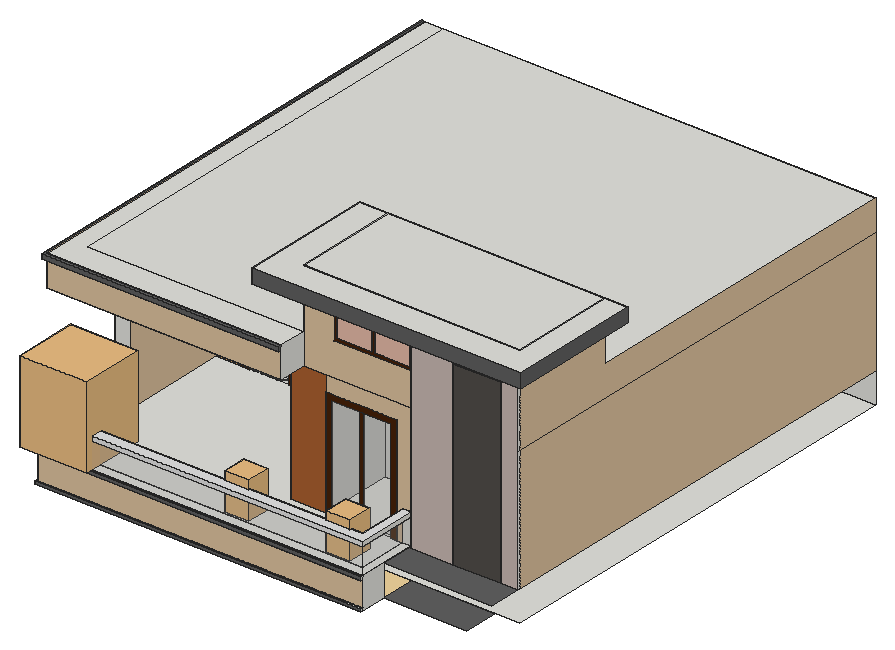
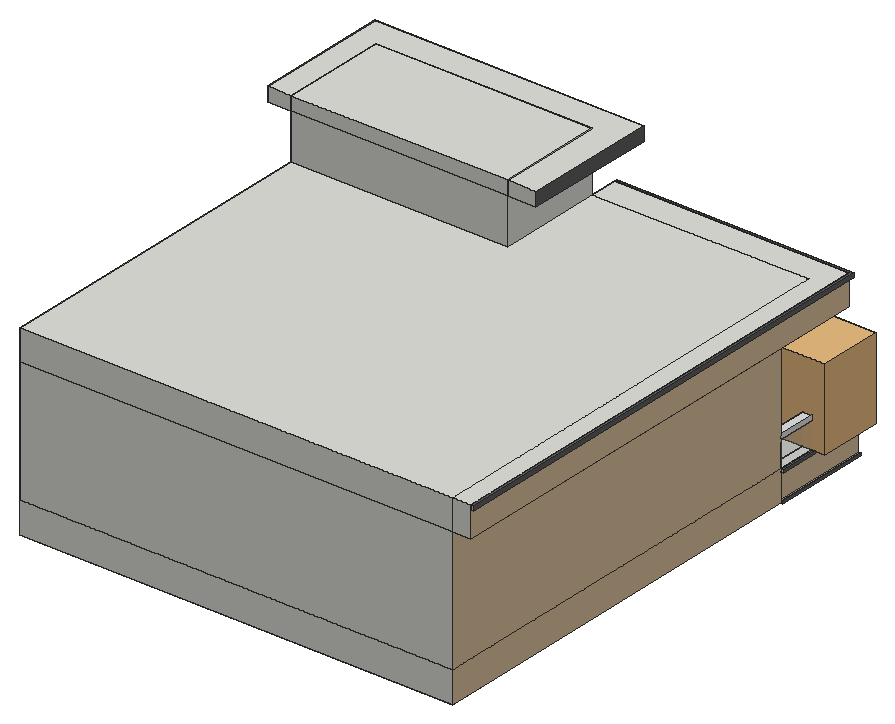
# SketchUp Ruby script. Lengths in inches.
U = 1.inch
M = Sketchup.active_model
def pt(a) = Geom::Point3d.new(a.map { |v| v * U })
def face(e, loops, mat)
  f = e.add_face(loops[0].map { |a| pt(a) })
  loops[1..].each { |l| e.add_face(l.map { |a| pt(a) }).erase! }
  f.material = f.back_material = mat if mat
  f
end
# faces: each face lists its corners as indices into pts; further lists are holes
def faces(e, pts, list, mat = nil) = list.each { |f| face(e, (f[0].is_a?(Array) ? f : [f]).map { |l| l.map { |i| pts[i] } }, mat) }
# xy, xz, yz: faces in a plane at the given z, y or x. An outline is a flat list of corners, or four numbers for a rectangle; further outlines are holes
def ring(l) = l.size == 4 ? [[l[0], l[1]], [l[2], l[1]], [l[2], l[3]], [l[0], l[3]]] : l.each_slice(2).to_a
def flat(e, list, mat, &to3) = list.each { |f| face(e, (f[0].is_a?(Array) ? f : [f]).map { |l| ring(l).map { |u, v| to3.(u, v) } }, mat) }
def xy(e, z, list, mat = nil) = flat(e, list, mat) { |x, y| [x, y, z] }
def xz(e, y, list, mat = nil) = flat(e, list, mat) { |x, z| [x, y, z] }
def yz(e, x, list, mat = nil) = flat(e, list, mat) { |y, z| [x, y, z] }
def lines(e, pts, list) = list.each { |a, b| e.add_line(pt(pts[a]), pt(pts[b])) }
# prism: a flat outline (further loops are holes) pulled along v
def prism(e, loops, v, mat = nil)
  f = face(e, loops, mat); d = Geom::Vector3d.new(v.map { |x| x * U })
  f.pushpull(f.normal.samedirection?(d) ? d.length : -d.length)
end
def box(e, o, s, mat = nil) = prism(e, [[o, [o[0] + s[0], o[1], o[2]], [o[0] + s[0], o[1] + s[1], o[2]], [o[0], o[1] + s[1], o[2]]]], [0, 0, s[2]], mat)
def at(x, y, z, deg = 0) = Geom::Transformation.translation(pt([x, y, z])) * Geom::Transformation.rotation(ORIGIN, Z_AXIS, deg.degrees)
def axes(o, x, y, z) = Geom::Transformation.new([*x, 0, *y, 0, *z, 0, *pt(o).to_a, 1])
def part(name) = M.definitions.add(name)
# library, detail: a bought-in or finely detailed component or shape, given as its bounding box
def library(name, o, s) = part(name).tap { |d| box(d.entities, o, s) }
def detail(e, o, s) = box(e.add_group.entities, o, s)
def put(e, d, t, mat = nil) = e.add_instance(d, t).tap { |i| i.material = mat if mat }
def group(e, t, mat = nil) = e.add_group.tap { |g| g.transformation = t; g.material = mat if mat }.entities
root = M.entities
M.materials.add("Generic").color = [222, 194, 159]
M.materials.add("Generic\#1").color = [230, 172, 103]
M.materials.add("Generic\#2").color = [241, 212, 157]
M.materials.add("[Color M01]").color = [226, 226, 226]
M.materials.add("[Color M07]").color = [96, 96, 96]
M.materials.add("[Mirror 02]").color = [229, 186, 167]
M.materials.add("[Roofing Shingles GAF Estates]").color = [81, 77, 74]
M.materials.add("[Stone Marble]").color = [201, 185, 179]
M.materials.add("[Translucent Glass Gray]").color = [175, 175, 175]
M.materials["[Translucent Glass Gray]"].alpha = 0.14
M.materials.add("[Wood Cherry Original]").color = [170, 96, 47]
M.materials.add("[Wood Veneer 01]").color = [71, 34, 9]
c1 = library("Group3\#1",[-238.15,54.18,0],[46.4,43.96,56.68])
c2 = part("Group\#3")
xy(c2.entities,0,[[0,0,140.875,6.8125]])
xy(c2.entities,105.3125,[[0,0,140.875,6.8125]])
xz(c2.entities,0,[[10.8,0,48.56,94.52],[52.56,0,88.32,94.52],[92.32,0,130.08,94.52]],"[Translucent Glass Gray]")
xz(c2.entities,0,[[0,0,10.8,0,10.8,94.52,48.56,94.52,48.56,0,52.56,0,52.56,94.52,88.32,94.52,88.32,0,92.32,0,92.32,94.52,130.08,94.52,130.08,0,140.875,0,140.875,105.3125,0,105.3125]],"[Wood Veneer 01]")
xz(c2.entities,6.8125,[[0,0,140.875,105.3125]],"[Translucent Glass Gray]")
yz(c2.entities,0,[[0,0,6.8125,105.3125]])
yz(c2.entities,140.875,[[0,0,6.8125,105.3125]])
c3 = library("Raised potted plant",[1.65,0,0],[13.63,13.63,20.73])
c4 = library("Tlon Light 450 Ceiling 152 006",[-8.86,-8.86,-3.78],[17.72,17.72,3.56])
xy(root,269.9375,[[217.875,91.73,217.875,228.48,35.6875,228.48,35.6875,125.1,20.1875,125.1,20.1875,523.73,440.1875,523.73,440.1875,91.73]])
xy(root,269.9375,[[[20.1875,32.23,20.1875,125.1,35.6875,125.1,35.6875,228.48,217.875,228.48,217.875,91.73,230.1875,91.73,230.1875,32.23],[58.88,55.42,194.68,205.29]],[230.1875,32.23,335.12,91.73]],"Generic\#2")
xy(root,269.9375,[[18.3125,30.41,18.3125,125.1,20.1875,125.1,20.1875,32.23,230.1875,32.23,230.1875,30.41],[230.1875,30.41,335.12,32.23],[335.12,57.98,416.1875,91.73]],"[Color M07]")
xy(root,269.9375,[[67.93,55.42,68.93,205.29],[78.5,55.42,79.5,205.29],[89.06,55.42,90.06,205.29],[99.62,55.42,100.62,205.29],[110.18,55.42,111.18,205.29],
  [120.75,55.42,121.75,205.29],[131.31,55.42,132.31,205.29],[141.87,55.42,142.87,205.29],[152.43,55.42,153.43,205.29],[163,55.42,164,205.29],
  [173.56,55.42,174.56,205.29],[184.12,55.42,185.12,205.29]],"[Wood Cherry Original]")
xy(root,272.5,[[230.1875,30.41,335.12,32.23]])
xy(root,272.5,[[18.3125,30.41,230.1875,30.41,230.1875,32.23,20.1875,32.23,20.1875,125.1,18.3125,125.1]],"[Color M07]")
xy(root,297,[[17.5625,30.41,17.5625,125.1,20.1875,125.1,20.1875,32.23,335.12,32.23,335.12,30.41]],"[Color M07]")
xy(root,299.875,[[20.1875,32.23,20.1875,125.1,29.125,125.1,29.125,42.6,326.8,42.6,326.8,91.73,335.12,91.73,335.12,32.23],[29.125,42.6,326.8,42.6,326.8,91.73,320.89,91.73,320.89,163.35,252.08,163.35,252.08,91.73,217.875,91.73,217.875,228.48,199.08,228.48,199.08,425.29,58.21,425.29,58.21,228.48,35.6875,228.48,35.6875,125.1,29.125,125.1],[337.01,89.1,377.69,91.73],[423.56,89.1,440.1875,91.73],[217.875,91.73,217.875,228.48,199.08,228.48,199.08,425.29,58.21,425.29,58.21,228.48,35.6875,228.48,35.6875,125.1,20.1875,125.1,20.1875,523.73,440.1875,523.73,440.1875,91.73,320.89,91.73,320.89,163.35,252.08,163.35,252.08,91.73]])
xy(root,299.875,[[17.5625,30.41,335.12,30.41,335.12,32.23,20.1875,32.23,20.1875,125.1,17.5625,125.1],[335.12,57.98,440.1875,57.98,440.1875,89.1,423.56,89.1,423.56,91.73,377.69,91.73,377.69,89.1,337.01,89.1,337.01,91.73,335.12,91.73]],"[Color M07]")
xy(root,325.25,[[20.1875,32.23,20.1875,125.1,29.125,125.1,29.125,42.6,326.8,42.6,326.8,91.73,335.12,91.73,335.12,32.23]])
xy(root,329.875,[[20.1875,32.23,335.12,32.23,335.12,91.73,326.8,91.73,326.8,42.6,29.125,42.6,29.125,125.1,20.1875,125.1]],"[Color M01]")
xy(root,404.625,[[252.08,91.73,320.89,163.35]])
xy(root,405.1875,[[58.21,228.48,199.08,425.29]])
xy(root,419.3125,[[52.42,86.71,65.86,206.5],[66.86,86.71,80.3125,206.5],[81.3125,86.71,94.76,206.5],[95.76,86.71,109.21,206.5],[110.21,86.71,123.66,206.5],
  [124.66,86.71,138.1,206.5],[139.1,86.71,152.55,206.5],[153.55,86.71,167,206.5],[168,86.71,181.45,206.5],[182.45,86.71,194.9,206.5]],"[Wood Cherry Original]")
xy(root,419.875,[[2.8125,228.48,20.1875,523.73]])
xy(root,419.875,[[[2.8125,64.73,2.8125,228.48,20.1875,228.48,20.1875,125.1,35.6875,125.1,35.6875,228.48,217.875,228.48,217.875,91.73,230.1875,91.73,230.1875,64.73],[52.42,86.71,194.9,206.5]]],"Generic\#2")
xy(root,419.875,[[65.86,86.71,66.86,206.5],[80.3125,86.71,81.3125,206.5],[94.76,86.71,95.76,206.5],[109.21,86.71,110.21,206.5],[123.66,86.71,124.66,206.5],
  [138.1,86.71,139.1,206.5],[152.55,86.71,153.55,206.5],[167,86.71,168,206.5],[181.45,86.71,182.45,206.5]],"[Wood Cherry Original]")
xy(root,445.25,[[0,64.73,2.8125,523.73]],"Generic")
xy(root,445.3125,[[0,61.91,230.1875,64.73]],"Generic")
xy(root,449.8125,[[2.8125,64.73,230.1875,64.73,230.1875,91.73,20.1875,91.73,20.1875,523.73,2.8125,523.73],[20.1875,91.73,230.1875,91.73,230.1875,194.66,440.1875,194.66,440.1875,523.73,20.1875,523.73]])
xy(root,449.8125,[[0,61.91,230.1875,61.91,230.1875,64.73,2.8125,64.73,2.8125,523.73,0,523.73]],"[Color M07]")
xy(root,455.39,[[262.97,91.73,296.69,119.1],[299.88,91.73,333.6,119.1]])
xy(root,474.97,[[377.69,89.1,423.56,91.73]])
xy(root,478.32,[[262.97,91.73,296.69,119.1],[299.88,91.73,333.6,119.1]])
xy(root,493.5625,[[337.01,89.1,440.1875,91.73],[230.1875,91.73,440.1875,194.66]])
xy(root,493.5625,[[202.5625,64.1,202.5625,194.66,230.1875,194.66,230.1875,91.73,337.01,91.73,337.01,89.1,440.1875,89.1,440.1875,194.66,462.9375,194.66,462.9375,64.1]],"[Wood Cherry Original]")
xy(root,507.375,[[202.5625,64.1,462.9375,64.1,462.9375,194.66,440.1875,194.66,440.1875,91.73,230.1875,91.73,230.1875,194.66,202.5625,194.66],[230.1875,91.73,440.1875,194.66]])
xz(root,30.41,[[18.3125,269.9375,335.12,272.5],[17.5625,297,335.12,299.875]],"[Color M07]")
xz(root,32.23,[[20.1875,269.9375,335.12,272.5],[20.1875,297,335.12,299.875]])
xz(root,32.23,[[20.1875,272.5,335.12,297]],"Generic")
xz(root,32.23,[[20.1875,325.25,335.12,329.875]],"[Color M01]")
xz(root,32.23,[[20.1875,299.875,335.12,325.25]],"[Translucent Glass Gray]")
xz(root,42.6,[[29.125,325.25,326.8,329.875]])
xz(root,42.6,[[29.125,299.875,326.8,325.25]],"[Translucent Glass Gray]")
xz(root,61.91,[[0,445.3125,230.1875,449.8125]],"[Color M07]")
xz(root,64.1,[[202.5625,493.5625,462.9375,507.375]],"[Color M07]")
xz(root,64.73,[[2.8125,419.875,230.1875,445.3125],[0,445.25,2.8125,445.3125],[2.8125,445.3125,230.1875,449.8125]],"Generic")
xz(root,86.71,[[52.42,419.3125,65.86,419.875],[66.86,419.3125,80.3125,419.875],[81.3125,419.3125,94.76,419.875],[95.76,419.3125,109.21,419.875],[110.21,419.3125,123.66,419.875],
  [124.66,419.3125,138.1,419.875],[139.1,419.3125,152.55,419.875],[153.55,419.3125,167,419.875],[168,419.3125,181.45,419.875],[182.45,419.3125,194.9,419.875]],"[Wood Cherry Original]")
xz(root,89.1,[[337.01,299.875,377.69,299.875,377.69,474.97,423.56,474.97,423.56,299.875,440.1875,299.875,440.1875,493.5625,337.01,493.5625]],"[Stone Marble]")
xz(root,91.73,[[326.8,299.875,335.12,325.25],[337.01,299.875,337.01,493.5625,440.1875,493.5625,440.1875,299.875,423.56,299.875,423.56,474.97,377.69,474.97,377.69,299.875],[377.69,299.875,423.56,474.97],[326.8,325.25,335.12,329.875],[230.1875,493.5625,440.1875,507.375]])
xz(root,91.73,[[320.89,299.875,326.8,299.875,326.8,329.875,335.12,329.875,335.12,299.875,337.01,299.875,337.01,419.875,252.08,419.875,252.08,404.625,320.89,404.625],[230.1875,419.875,337.01,419.875,337.01,451.98,259.5625,451.98,259.5625,481.73,337.01,481.73,337.01,493.5625,230.1875,493.5625]],"Generic")
xz(root,91.73,[[262.97,455.39,296.69,478.32],[299.88,455.39,333.6,478.32]],"[Mirror 02]")
xz(root,91.73,[[217.875,299.875,252.08,419.875]],"[Wood Cherry Original]")
xz(root,91.73,[[[259.5625,451.98,337.01,481.73],[299.88,455.39,333.6,478.32],[262.97,455.39,296.69,478.32]]],"[Wood Veneer 01]")
xz(root,119.1,[[262.97,455.39,296.69,478.32],[299.88,455.39,333.6,478.32]])
xz(root,125.1,[[18.3125,269.9375,20.1875,272.5],[17.5625,297,20.1875,299.875],[29.125,299.875,35.6875,299.875,35.6875,419.875,20.1875,419.875,20.1875,329.875,29.125,329.875]])
xz(root,163.35,[[252.08,299.875,320.89,404.625]])
xz(root,194.66,[[230.1875,449.8125,440.1875,493.5625],[202.5625,493.5625,230.1875,507.375],[230.1875,493.5625,440.1875,507.375],[440.1875,493.5625,462.9375,507.375]])
xz(root,206.5,[[52.42,419.3125,65.86,419.875],[66.86,419.3125,80.3125,419.875],[81.3125,419.3125,94.76,419.875],[95.76,419.3125,109.21,419.875],[110.21,419.3125,123.66,419.875],
  [124.66,419.3125,138.1,419.875],[139.1,419.3125,152.55,419.875],[153.55,419.3125,167,419.875],[168,419.3125,181.45,419.875],[182.45,419.3125,194.9,419.875]])
xz(root,228.48,[[35.6875,299.875,58.21,299.875,58.21,405.1875,199.08,405.1875,199.08,299.875,217.875,299.875,217.875,419.875,35.6875,419.875]],"Generic\#1")
xz(root,425.29,[[58.21,299.875,199.08,405.1875]])
xz(root,523.73,[[20.1875,269.9375,440.1875,299.875],[20.1875,299.875,440.1875,419.875],[2.8125,419.875,20.1875,449.8125],[20.1875,419.875,440.1875,449.8125]])
xz(root,523.73,[[0,445.25,2.8125,449.8125]],"Generic")
yz(root,0,[[64.73,445.25,64.73,445.3125,61.91,445.3125,61.91,449.8125,523.73,449.8125,523.73,445.25]],"[Color M07]")
yz(root,2.8125,[[64.73,419.875,523.73,445.25],[64.73,445.25,523.73,449.8125]],"Generic")
yz(root,17.5625,[[30.41,297,125.1,299.875]],"[Color M07]")
yz(root,18.3125,[[30.41,269.9375,125.1,272.5]],"[Color M07]")
yz(root,20.1875,[[32.23,269.9375,125.1,272.5],[32.23,297,125.1,299.875]])
yz(root,20.1875,[[125.1,269.9375,523.73,299.875],[32.23,272.5,125.1,297],[125.1,299.875,523.73,419.875]],"Generic")
yz(root,20.1875,[[32.23,325.25,125.1,329.875]],"[Color M01]")
yz(root,20.1875,[[32.23,299.875,125.1,325.25]],"[Translucent Glass Gray]")
yz(root,29.125,[[42.6,325.25,125.1,329.875]])
yz(root,29.125,[[42.6,299.875,125.1,325.25]],"[Translucent Glass Gray]")
yz(root,35.6875,[[125.1,299.875,228.48,419.875]],"Generic")
yz(root,52.42,[[86.71,419.3125,103.12,419.875],[103.12,419.3125,206.5,419.875]],"[Wood Cherry Original]")
yz(root,58.21,[[228.48,299.875,425.29,405.1875]])
yz(root,65.86,[[86.71,419.3125,206.5,419.875]],"[Wood Cherry Original]")
yz(root,66.86,[[86.71,419.3125,206.5,419.875]],"[Wood Cherry Original]")
yz(root,80.3125,[[86.71,419.3125,206.5,419.875]],"[Wood Cherry Original]")
yz(root,81.3125,[[86.71,419.3125,206.5,419.875]],"[Wood Cherry Original]")
yz(root,94.76,[[86.71,419.3125,206.5,419.875]],"[Wood Cherry Original]")
yz(root,95.76,[[86.71,419.3125,206.5,419.875]],"[Wood Cherry Original]")
yz(root,109.21,[[86.71,419.3125,206.5,419.875]],"[Wood Cherry Original]")
yz(root,110.21,[[86.71,419.3125,206.5,419.875]],"[Wood Cherry Original]")
yz(root,123.66,[[86.71,419.3125,206.5,419.875]],"[Wood Cherry Original]")
yz(root,124.66,[[86.71,419.3125,206.5,419.875]],"[Wood Cherry Original]")
yz(root,138.1,[[86.71,419.3125,206.5,419.875]],"[Wood Cherry Original]")
yz(root,139.1,[[86.71,419.3125,206.5,419.875]],"[Wood Cherry Original]")
yz(root,152.55,[[86.71,419.3125,206.5,419.875]],"[Wood Cherry Original]")
yz(root,153.55,[[86.71,419.3125,206.5,419.875]],"[Wood Cherry Original]")
yz(root,167,[[86.71,419.3125,206.5,419.875]],"[Wood Cherry Original]")
yz(root,168,[[86.71,419.3125,206.5,419.875]],"[Wood Cherry Original]")
yz(root,181.45,[[86.71,419.3125,206.5,419.875]],"[Wood Cherry Original]")
yz(root,182.45,[[86.71,419.3125,206.5,419.875]],"[Wood Cherry Original]")
yz(root,194.9,[[86.71,419.3125,206.5,419.875]],"[Wood Cherry Original]")
yz(root,199.08,[[228.48,299.875,425.29,405.1875]])
yz(root,202.5625,[[64.1,493.5625,194.66,507.375]],"[Color M07]")
yz(root,217.875,[[91.73,299.875,228.48,419.875]],"[Wood Cherry Original]")
yz(root,230.1875,[[64.73,419.875,91.73,449.8125],[91.73,449.8125,194.66,493.5625],[91.73,493.5625,194.66,507.375]])
yz(root,230.1875,[[61.91,445.3125,64.73,449.8125]],"[Color M07]")
yz(root,252.08,[[91.73,299.875,163.35,404.625]])
yz(root,262.97,[[91.73,455.39,119.1,478.32]])
yz(root,296.69,[[91.73,455.39,119.1,478.32]])
yz(root,299.88,[[91.73,455.39,119.1,478.32]])
yz(root,320.89,[[91.73,299.875,163.35,404.625]])
yz(root,326.8,[[42.6,325.25,91.73,329.875]])
yz(root,326.8,[[42.6,299.875,91.73,325.25]],"[Translucent Glass Gray]")
yz(root,333.6,[[91.73,455.39,119.1,478.32]])
yz(root,335.12,[[30.41,269.9375,32.23,272.5],[32.23,269.9375,57.98,299.875],[30.41,297,32.23,299.875],[32.23,325.25,91.73,329.875]])
yz(root,335.12,[[32.23,299.875,91.73,325.25]],"[Translucent Glass Gray]")
yz(root,337.01,[[89.1,299.875,91.73,493.5625]])
yz(root,377.69,[[89.1,299.875,91.73,474.97]])
yz(root,423.56,[[89.1,299.875,91.73,474.97]])
yz(root,440.1875,[[89.1,299.875,91.73,419.875],[89.1,419.875,91.73,493.5625],[91.73,493.5625,194.66,507.375]])
yz(root,440.1875,[[91.73,299.875,523.73,419.875],[91.73,419.875,523.73,419.875,523.73,449.8125,194.66,449.8125,194.66,493.5625,91.73,493.5625]],"Generic")
yz(root,462.9375,[[64.1,493.5625,194.66,507.375]],"[Color M07]")
g1 = group(root,at(194.68,55.42,269.9375))
p = [[0,13.12,0],[0,0,0],[0,149.87,0]]
lines(g1,p,[[0,1],[2,0]])
put(root,c1,axes([341.34,-49.71,299.875],[1.4025,0,0],[0,1.4025,0],[0,0,1.4025]))
g2 = group(root,at(252.08,91.73,299.875))
xy(g2,0,[[0,0,68.8125,2.8125]])
xy(g2,104.75,[[0,0,68.8125,2.8125]])
xz(g2,0,[[5.83,0,32.41,98.92],[36.41,0,62.98,98.92]],"[Translucent Glass Gray]")
xz(g2,0,[[0,0,5.83,0,5.83,98.92,62.98,98.92,62.98,0,68.8125,0,68.8125,104.75,0,104.75],[32.41,0,36.41,98.92]],"[Wood Veneer 01]")
xz(g2,2.8125,[[0,0,68.8125,104.75]],"[Translucent Glass Gray]")
yz(g2,0,[[0,0,2.8125,104.75]])
yz(g2,68.8125,[[0,0,2.8125,104.75]])
put(root,c2,at(58.21,228.48,299.875))
g3 = group(root,at(377.69,89.1,299.875))
xz(g3,0,[[0,0,45.86,175.09]],"[Roofing Shingles GAF Estates]")
put(root,c3,axes([289.42,41.7,302.11],[1.72,0,0],[0,1.72,0],[0,0,1.72]))
put(root,c3,axes([190.73,41.7,302.11],[1.72,0,0],[0,1.72,0],[0,0,1.72]))
put(root,c4,axes([74.4375,109.77,419.42],[0.5,0,0],[0,0.5,0],[0,0,0.5]))
put(root,c4,axes([74.4375,170.14,419.42],[0.5,0,0],[0,0.5,0],[0,0,0.5]))
put(root,c4,axes([117.5,109.77,419.42],[0.5,0,0],[0,0.5,0],[0,0,0.5]))
put(root,c4,axes([117.5,170.14,419.42],[0.5,0,0],[0,0.5,0],[0,0,0.5]))
put(root,c4,axes([160.5625,109.77,419.42],[0.5,0,0],[0,0.5,0],[0,0,0.5]))
put(root,c4,axes([160.5625,170.14,419.42],[0.5,0,0],[0,0.5,0],[0,0,0.5]))
put(root,c4,axes([415.75,76.37,494.02],[0.5,0,0],[0,0.5,0],[0,0,0.5]))
put(root,c4,axes([384.37,76.37,494.02],[0.5,0,0],[0,0.5,0],[0,0,0.5]))
put(root,c4,axes([353,76.37,494.02],[0.5,0,0],[0,0.5,0],[0,0,0.5]))
put(root,c4,axes([321.62,76.37,494.02],[0.5,0,0],[0,0.5,0],[0,0,0.5]))
put(root,c4,axes([284.18,76.37,494.02],[0.5,0,0],[0,0.5,0],[0,0,0.5]))
put(root,c4,axes([246.75,76.37,494.02],[0.5,0,0],[0,0.5,0],[0,0,0.5]))
